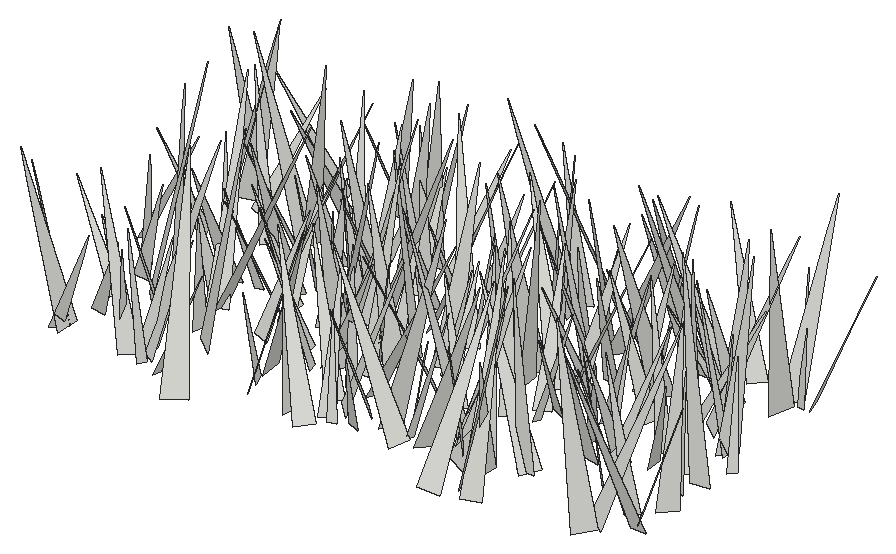
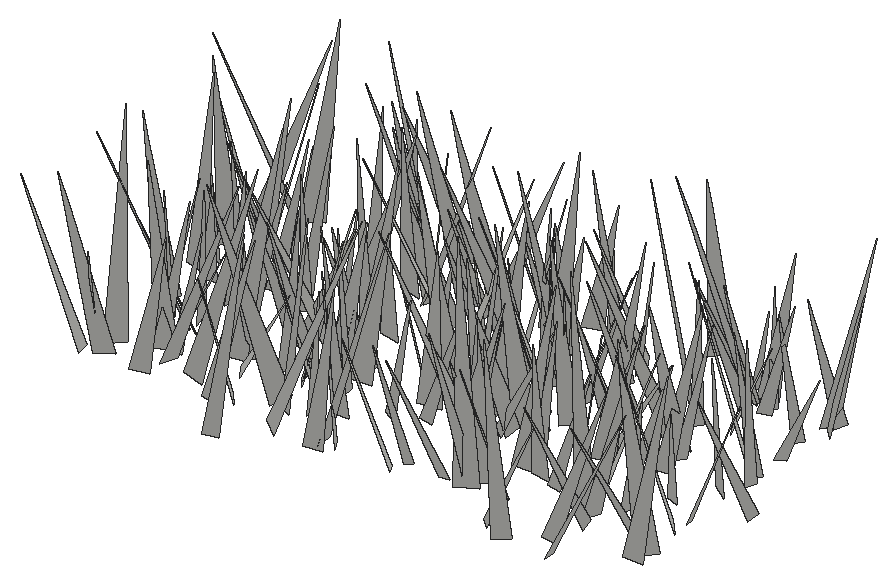
# SketchUp Ruby script. Lengths in inches.
U = 1.inch
M = Sketchup.active_model
def pt(a) = Geom::Point3d.new(a.map { |v| v * U })
def face(e, loops, mat)
  f = e.add_face(loops[0].map { |a| pt(a) })
  loops[1..].each { |l| e.add_face(l.map { |a| pt(a) }).erase! }
  f.material = f.back_material = mat if mat
  f
end
# faces: each face lists its corners as indices into pts; further lists are holes
def faces(e, pts, list, mat = nil) = list.each { |f| face(e, (f[0].is_a?(Array) ? f : [f]).map { |l| l.map { |i| pts[i] } }, mat) }
# xy, xz, yz: faces in a plane at the given z, y or x. An outline is a flat list of corners, or four numbers for a rectangle; further outlines are holes
def ring(l) = l.size == 4 ? [[l[0], l[1]], [l[2], l[1]], [l[2], l[3]], [l[0], l[3]]] : l.each_slice(2).to_a
def flat(e, list, mat, &to3) = list.each { |f| face(e, (f[0].is_a?(Array) ? f : [f]).map { |l| ring(l).map { |u, v| to3.(u, v) } }, mat) }
def xy(e, z, list, mat = nil) = flat(e, list, mat) { |x, y| [x, y, z] }
def xz(e, y, list, mat = nil) = flat(e, list, mat) { |x, z| [x, y, z] }
def yz(e, x, list, mat = nil) = flat(e, list, mat) { |y, z| [x, y, z] }
def lines(e, pts, list) = list.each { |a, b| e.add_line(pt(pts[a]), pt(pts[b])) }
# prism: a flat outline (further loops are holes) pulled along v
def prism(e, loops, v, mat = nil)
  f = face(e, loops, mat); d = Geom::Vector3d.new(v.map { |x| x * U })
  f.pushpull(f.normal.samedirection?(d) ? d.length : -d.length)
end
def box(e, o, s, mat = nil) = prism(e, [[o, [o[0] + s[0], o[1], o[2]], [o[0] + s[0], o[1] + s[1], o[2]], [o[0], o[1] + s[1], o[2]]]], [0, 0, s[2]], mat)
def at(x, y, z, deg = 0) = Geom::Transformation.translation(pt([x, y, z])) * Geom::Transformation.rotation(ORIGIN, Z_AXIS, deg.degrees)
def axes(o, x, y, z) = Geom::Transformation.new([*x, 0, *y, 0, *z, 0, *pt(o).to_a, 1])
def part(name) = M.definitions.add(name)
# library, detail: a bought-in or finely detailed component or shape, given as its bounding box
def library(name, o, s) = part(name).tap { |d| box(d.entities, o, s) }
def detail(e, o, s) = box(e.add_group.entities, o, s)
def put(e, d, t, mat = nil) = e.add_instance(d, t).tap { |i| i.material = mat if mat }
def group(e, t, mat = nil) = e.add_group.tap { |g| g.transformation = t; g.material = mat if mat }.entities
root = M.entities
c1 = part("fur_instance\#9")
p = [[0.8125,0,1.79],[0.67,-0.02,1.48],[0,-0.11,0],[0,0.11,0]]
faces(c1.entities,p,[[0,1,2,3]])
put(root,c1,axes([504.47,355.8125,-21.66],[-6.49711,1.14641,2.18071],[1.63194,6.61021,1.38712],[1.84567,-1.80917,6.45001]))
put(root,c1,axes([515.51,352.76,-21.66],[-5.56313,6.05819,1.00831],[6.02083,5.64819,-0.71719],[1.2116,-0.25113,8.19364]))
put(root,c1,axes([503.92,355.33,-21.66],[3.45367,-2.54495,0.42724],[-2.57712,-3.36456,0.79082],[0.1334,0.88889,4.21654]))
put(root,c1,axes([546.35,355.52,-21.66],[-5.45216,4.70878,2.71596],[5.23215,5.58914,0.81316],[1.47433,-2.42158,7.15803]))
put(root,c1,axes([512.55,354.71,-21.66],[3.9235,0.14114,0.37721],[0.06723,-3.8717,0.74932],[-0.3971,0.73898,3.85386]))
put(root,c1,axes([508.625,356.28,-21.66],[3.85883,-1.0172,1.02296],[-0.87371,-3.97244,-0.65425],[-1.14794,-0.39587,3.93665]))
put(root,c1,axes([526.52,357.02,-21.66],[-0.43336,-3.79274,0.22877],[-3.61563,0.48241,1.14868],[1.16807,0.08612,3.64049]))
put(root,c1,axes([536.4,355.625,-21.66],[7.04246,3.4796,1.7186],[3.70112,-7.09298,-0.80545],[-1.16744,-1.49647,7.81378]))
put(root,c1,axes([509.68,355.46,-21.66],[-3.34146,5.15286,1.47209],[5.35695,3.16362,1.08579],[-0.14849,-1.82317,6.0447]))
put(root,c1,axes([535.42,353.48,-21.66],[-1.59566,7.05244,0.57454],[6.94745,1.67322,-1.24356],[1.34162,-0.27674,7.12297]))
put(root,c1,axes([548.9,357.82,-21.66],[-1.75901,-6.72397,0.92553],[-6.70142,1.56883,-1.33876],[-1.07676,1.22044,6.82009]))
put(root,c1,axes([510.99,355.13,-21.66],[-4.31173,0.11749,0.33288],[0.02447,4.16916,-1.1546],[0.35215,1.14887,4.15592]))
put(root,c1,axes([504.12,356.31,-21.66],[-4.01169,-3.78695,1.3287],[-4.00574,3.89344,-0.9976],[0.2459,1.64323,5.42581]))
put(root,c1,axes([536.8,357.75,-21.66],[4.83805,-1.95602,0.87332],[-1.75837,-4.85831,-1.14034],[-1.22345,-0.75248,5.09238]))
put(root,c1,axes([522.14,355.82,-21.66],[-3.8319,-0.08961,1.0116],[-0.27638,3.8917,-0.7022],[0.97723,0.7493,3.76807]))
put(root,c1,axes([524.01,355.26,-21.66],[-3.78417,5.30239,0.2634],[5.25954,3.70033,1.07214],[-0.72248,-0.83479,6.42541]))
put(root,c1,axes([510.1875,356.3125,-21.66],[0.83525,-3.69964,2.10924],[-4.22949,-0.46947,0.8514],[0.49764,2.21949,3.69595]))
put(root,c1,axes([508.67,357.04,-21.66],[-2.76713,3.18046,1.2921],[3.43249,2.58898,0.97827],[0.05304,-1.61979,4.10065]))
put(root,c1,axes([534.81,357.94,-21.66],[3.60771,1.96245,2.32029],[2.67745,-3.75626,-0.98607],[-1.43745,-2.07119,3.98679]))
put(root,c1,axes([518.16,357.95,-21.66],[-3.2792,-1.26365,1.37089],[-0.97388,3.52607,0.9207],[1.58988,-0.44645,3.3915]))
put(root,c1,axes([530.21,357.05,-21.66],[-6.66331,2.16551,0.21128],[2.17487,6.60915,0.85019],[-0.06344,-0.87375,6.95459]))
put(root,c1,axes([526.24,359.1,-21.66],[-3.04266,-3.74721,0.50143],[-3.60797,3.07034,1.05183],[1.12942,-0.28668,4.71094]))
put(root,c1,axes([538.24,354.21,-21.66],[0.0768,8.17284,0.16546],[8.06568,-0.10268,1.32775],[-1.3295,-0.15078,8.06464]))
put(root,c1,axes([510.43,356.23,-21.66],[4.03025,7.20792,1.49357],[7.34455,-3.82368,-1.36555],[0.49235,-1.96292,8.14446]))
put(root,c1,axes([504.72,358.59,-21.66],[1.3305,-3.93215,0.09517],[-3.71952,-1.22514,1.38031],[1.27907,0.52755,3.91494]))
put(root,c1,axes([531.71,357.85,-21.66],[6.48225,-3.39085,0.68777],[-3.4557,-6.41712,0.9323],[-0.17042,1.14593,7.25591]))
put(root,c1,axes([525.15,356.56,-21.66],[-0.19051,3.61425,0.52762],[3.57644,0.0773,0.76192],[-0.74175,-0.55561,3.53816]))
put(root,c1,axes([534.33,357.69,-21.66],[1.01992,4.1189,1.46608],[4.23417,-0.55549,-1.38501],[1.0893,-1.69737,4.0109]))
put(root,c1,axes([510.3,357.03,-21.66],[3.86814,-0.78573,1.02615],[-1.07279,-3.75781,1.16655],[-0.72076,1.37634,3.77081]))
put(root,c1,axes([546.43,359.55,-21.66],[-4.48519,-3.52054,0.94744],[-3.42145,4.58335,0.83384],[1.25916,-0.08621,5.64055]))
put(root,c1,axes([518.52,356.51,-21.66],[4.75922,3.00167,0.77273],[2.8511,-4.79497,1.06623],[-1.21588,0.50555,5.5248]))
put(root,c1,axes([517.86,359.57,-21.66],[6.9866,-0.46387,0.39437],[-0.38095,-6.874,-1.33651],[-0.47495,-1.31005,6.87325]))
put(root,c1,axes([524.48,356.93,-21.66],[-3.96377,3.38106,0.80717],[3.27975,4.04327,-0.83051],[1.15166,0.12228,5.14327]))
put(root,c1,axes([533.98,358.76,-21.66],[4.85202,-3.37562,1.03104],[-3.52041,-4.75453,1.00059],[-0.25408,1.41409,5.82544]))
put(root,c1,axes([546.23,356.82,-21.66],[3.64323,6.95762,0.66244],[6.95502,-3.53547,-1.11744],[0.68929,-1.10109,7.77386]))
put(root,c1,axes([548.1,359.01,-21.66],[4.88732,1.92922,0.49219],[1.99044,-4.76555,-1.08522],[-0.04774,-1.19066,5.14102]))
put(root,c1,axes([524.73,358.3125,-21.66],[4.20289,4.66758,0.96744],[4.74909,-3.98911,-1.38552],[0.41036,-1.63927,6.12625]))
put(root,c1,axes([534.64,357.26,-21.66],[3.51205,7.24819,1.1392],[7.33442,-3.43356,-0.76524],[0.20101,-1.35755,8.01781]))
put(root,c1,axes([534.61,358.64,-21.66],[-7.94923,-1.56442,0.5472],[-1.62855,7.87073,-1.15603],[0.30767,1.24144,8.0188]))
put(root,c1,axes([547.24,359.23,-21.66],[0.3865,-5.10308,2.42648],[-5.49086,-0.91339,-1.04632],[-1.33405,2.28099,5.00959]))
put(root,c1,axes([529.2,359.67,-21.66],[3.2608,1.42212,0.87051],[1.60342,-3.19897,-0.78016],[-0.45742,-1.07574,3.47082]))
put(root,c1,axes([530.23,358.1,-21.66],[4.26964,0.47793,1.18834],[0.14194,-4.28676,1.21405],[-1.27296,1.12502,4.1212]))
put(root,c1,axes([528.43,358.43,-21.66],[7.3545,-2.24014,2.18394],[-2.66673,-7.40612,1.38362],[-1.63595,2.00191,7.56257]))
put(root,c1,axes([538.65,359.22,-21.66],[-1.16984,-6.03511,2.92768],[-6.70455,0.96018,-0.69968],[-0.2073,3.00298,6.1075]))
put(root,c1,axes([538.87,359.4,-21.66],[-5.22041,4.31379,0.87725],[4.39805,5.05275,1.32586],[-0.18846,-1.57859,6.64105]))
put(root,c1,axes([512.71,359.26,-21.66],[4.94057,6.27292,2.28459],[6.62263,-4.9638,-0.69253],[-0.84236,-2.23369,7.95482]))
put(root,c1,axes([511.12,360.8125,-21.66],[4.3252,-1.84495,1.08949],[-1.74272,-4.45705,-0.62914],[-1.2465,-0.1704,4.65998]))
put(root,c1,axes([523.49,358.92,-21.66],[-3.54308,4.52564,0.44169],[4.5332,3.47169,0.79207],[-0.35583,-0.83417,5.69276]))
put(root,c1,axes([544.8,359.54,-21.66],[-3.71707,-2.68533,1.32909],[-2.9797,3.53518,-1.19076],[0.31439,1.75658,4.42828]))
put(root,c1,axes([509.03,359.91,-21.66],[-3.56795,-1.90054,0.20659],[-1.88749,3.43261,-1.0196],[-0.30353,0.99505,3.91187]))
put(root,c1,axes([535.87,358.77,-21.66],[0.42916,7.00561,1.64499],[7.11073,-0.66598,0.98114],[-1.10544,-1.56418,6.94983]))
put(root,c1,axes([521.37,362.57,-21.66],[4.41778,-6.32124,1.65754],[-6.32459,-4.6393,-0.83587],[-1.6447,0.86086,7.66656]))
put(root,c1,axes([540.92,362.95,-21.66],[-0.50575,-5.47671,0.42869],[-5.44927,0.55465,0.65709],[0.69543,0.36321,5.46062]))
put(root,c1,axes([504.24,361.02,-21.66],[-3.16167,2.60611,0.16715],[2.5519,3.02748,1.0668],[-0.55458,-0.92652,3.956]))
put(root,c1,axes([527.65,364.02,-21.66],[-3.98509,-5.15803,0.00595],[-5.07141,3.91953,1.18509],[0.94137,-0.71992,6.40951]))
put(root,c1,axes([519.8,361.34,-21.66],[-5.05494,-2.22544,0.30278],[-2.23904,4.935,-1.10864],[-0.17591,1.1357,5.41072]))
put(root,c1,axes([525.05,361,-21.66],[6.85637,-0.90607,0.05149],[-0.90407,-6.7849,0.99057],[0.07926,0.98874,6.84468]))
put(root,c1,axes([548.83,360.82,-21.66],[5.64429,-3.09602,3.33103],[-3.78051,-6.14532,0.69416],[-2.52761,2.27789,6.40012]))
put(root,c1,axes([520.56,362.1,-21.66],[4.45339,-2.56263,0.11815],[-2.55046,-4.39735,0.75645],[0.27609,0.71411,5.08208]))
put(root,c1,axes([518.36,362.95,-21.66],[-4.47409,-0.55232,0.95951],[-0.288,4.43762,1.21151],[1.069,-1.11608,4.34221]))
put(root,c1,axes([521.87,363.01,-21.66],[-2.90046,-3.39812,1.38689],[-3.27993,3.19309,0.96417],[1.64705,0.37459,4.36237]))
put(root,c1,axes([523.17,361.1,-21.66],[-4.45117,0.87592,1.04433],[0.68712,4.52233,-0.86441],[1.17717,0.67238,4.45342]))
put(root,c1,axes([542.72,363.91,-21.66],[2.25117,-4.50739,0.41367],[-4.42833,-2.28883,-0.84056],[-0.93676,-0.01195,4.96767]))
put(root,c1,axes([530.92,360.55,-21.66],[-2.87102,4.68172,0.40163],[4.57171,2.89185,-1.02921],[1.08596,0.20316,5.39463]))
put(root,c1,axes([504.1,363.71,-21.66],[1.4923,-4.43759,0.64343],[-4.35505,-1.27294,1.3215],[1.06759,1.01025,4.49142]))
put(root,c1,axes([521.22,361.35,-21.66],[7.46967,2.68884,2.29218],[2.3982,-7.79505,1.32883],[-2.59473,0.53597,7.82688]))
put(root,c1,axes([514.8,362.32,-21.66],[0.90877,4.85728,1.17196],[4.86719,-0.59112,-1.32422],[1.13009,-1.36012,4.76083]))
put(root,c1,axes([539.5,364.69,-21.66],[4.03439,-1.67825,0.01541],[-1.64329,-3.95818,-0.85174],[-0.3411,-0.78061,4.28572]))
put(root,c1,axes([544.43,364.96,-21.66],[4.66467,-0.77947,0.02704],[-0.7406,-4.47818,-1.32848],[-0.24456,-1.30606,4.53893]))
put(root,c1,axes([522.87,364.08,-21.66],[4.02483,1.17033,1.17041],[1.40502,-4.04247,-0.78939],[-0.87491,-1.10794,4.11653]))
put(root,c1,axes([542.56,362.9,-21.66],[2.02103,5.13059,0.73898],[5.12624,-1.86067,-1.10143],[0.76856,-1.08099,5.40318]))
put(root,c1,axes([503.64,364.75,-21.66],[4.65785,-0.69082,1.21899],[-0.53967,-4.78978,-0.65231],[-1.29303,-0.48941,4.6634]))
put(root,c1,axes([547.98,363.13,-21.66],[1.43677,3.63281,1.03111],[3.57622,-1.66329,0.8769],[-1.21291,-0.60083,3.80693]))
put(root,c1,axes([523.82,364.66,-21.66],[4.51203,-4.20905,2.90182],[-4.30887,-5.21386,-0.8628],[-2.75143,1.26279,6.10984]))
put(root,c1,axes([509.2,364.93,-21.66],[-4.57691,0.82768,1.57562],[1.18388,4.66198,0.99001],[1.32893,-1.30255,4.54457]))
put(root,c1,axes([530.36,363.13,-21.66],[-1.14245,4.14217,0.46464],[4.01441,0.96381,1.27839],[-1.12161,-0.76952,4.10226]))
put(root,c1,axes([530.07,361.83,-21.66],[5.64336,5.1887,0.30355],[5.15395,-5.64438,0.66329],[-0.67191,0.28398,7.63742]))
put(root,c1,axes([506.14,362.1,-21.66],[-5.10797,-4.03263,5.02727],[-5.71036,5.80586,-1.14484],[2.98787,4.202,6.40647]))
put(root,c1,axes([519.36,363.625,-21.66],[-4.01098,-1.65554,1.8183],[-2.11594,4.09606,-0.93811],[1.25294,1.61753,4.23659]))
put(root,c1,axes([509.04,366.8,-21.66],[1.9027,-5.40071,0.1352],[-5.35593,-1.9045,-0.70218],[-0.70705,-0.10684,5.68285]))
put(root,c1,axes([535.49,366.47,-21.66],[-0.82646,-4.24361,0.01629],[-4.06802,0.79698,1.2278],[1.20816,-0.21938,4.14533]))
put(root,c1,axes([519.57,365.82,-21.66],[4.8829,2.83209,2.83107],[3.60518,-5.05239,-1.16384],[-1.7431,-2.51617,5.52349]))
put(root,c1,axes([510.49,363.76,-21.66],[7.61599,0.93725,0.32253],[0.89381,-7.57423,0.90437],[-0.42844,0.85927,7.61996]))
put(root,c1,axes([523.23,362.58,-21.66],[1.19903,6.87384,0.5978],[6.78552,-1.2847,1.16229],[-1.25048,-0.38022,6.88014]))
put(root,c1,axes([517.38,365.77,-21.66],[3.13574,-5.33007,1.5739],[-5.55752,-3.01682,0.85589],[-0.02918,1.79133,6.12454]))
put(root,c1,axes([548.32,364.73,-21.66],[-0.94907,-6.99906,3.73248],[-7.88487,0.42284,-1.21201],[-0.8643,3.82797,6.95835]))
put(root,c1,axes([527.21,365.42,-21.66],[1.77196,3.84512,1.4323],[4.08534,-1.50774,-1.0065],[0.38272,-1.70823,4.11239]))
put(root,c1,axes([513.53,365.76,-21.66],[-2.7685,-2.84273,0.0732],[-2.6967,2.59213,-1.32656],[-0.90237,0.97511,3.73978]))
put(root,c1,axes([512.94,368.01,-21.66],[2.89826,-6.60565,0.55734],[-6.55377,-2.94663,-0.84295],[-0.99662,0.16719,7.16407]))
put(root,c1,axes([513.47,364.89,-21.66],[4.56915,3.9518,0.34933],[3.96081,-4.51383,-0.74378],[0.22516,-0.79028,5.99505]))
put(root,c1,axes([533.29,364.11,-21.66],[-0.40472,6.25604,0.83945],[6.18781,0.22712,1.29072],[-1.24649,-0.90382,6.13481]))
put(root,c1,axes([535.0625,364.87,-21.66],[3.77133,0.16267,0.95437],[-0.10228,-3.74984,1.04331],[-0.96272,1.03561,3.6278]))
put(root,c1,axes([514.96,364.61,-21.66],[-0.69382,4.82103,0.91338],[4.82167,0.84094,-0.77604],[0.90996,-0.78004,4.80848]))
put(root,c1,axes([514.3125,366.68,-21.66],[-4.64353,0.24048,0.81476],[0.40253,4.60984,0.93348],[0.74809,-0.98772,4.55508]))
put(root,c1,axes([541.4375,364.29,-21.66],[1.45734,4.18221,0.34787],[4.02467,-1.49715,1.13854],[-1.18907,0.05834,4.28]))
put(root,c1,axes([510.81,367.19,-21.66],[-0.75955,-3.70224,0.74684],[-3.72635,0.61048,-0.76351],[-0.61539,0.87293,3.70143]))
put(root,c1,axes([510.29,363.62,-21.66],[-0.64935,7.68845,0.01437],[7.6155,0.6412,1.06165],[-1.05669,-0.10353,7.64243]))
put(root,c1,axes([546.79,365.46,-21.66],[-1.86757,4.60063,0.33127],[4.58089,1.80817,0.71369],[-0.53944,-0.57279,4.91369]))
put(root,c1,axes([524.35,366.22,-21.66],[-6.69372,-1.63538,1.73187],[-1.91789,6.76382,-1.02573],[1.41263,1.43387,6.81383]))
put(root,c1,axes([520.12,364.43,-21.66],[5.47327,5.90798,0.9862],[5.7796,-5.55993,1.23167],[-1.57262,0.12835,7.95889]))
put(root,c1,axes([526.42,366.43,-21.66],[-2.68799,6.56885,2.98447],[6.8694,3.30396,-1.08507],[2.20641,-2.2839,7.01411]))
put(root,c1,axes([518.26,366.83,-21.66],[4.16572,3.95636,0.93283],[4.06431,-4.03236,-1.04767],[0.06588,-1.40123,5.64875]))
put(root,c1,axes([531.66,368.18,-21.66],[7.52805,-0.18805,1.99939],[0.07054,-7.72753,-0.99239],[-2.00698,-0.97696,7.46472]))
put(root,c1,axes([543.89,366.61,-21.66],[-5.59826,1.4556,0.99849],[1.35798,5.67289,-0.65612],[1.12768,0.39476,5.74707]))
put(root,c1,axes([537,368.57,-21.66],[-0.83843,-4.56243,0.7415],[-4.45874,0.59959,-1.35228],[-1.2187,0.94513,4.43735]))
put(root,c1,axes([534.55,366.07,-21.66],[-3.134,4.47853,0.59876],[4.43295,3.18866,-0.64743],[0.8745,-0.1137,5.42771]))
put(root,c1,axes([504.61,366.59,-21.66],[2.34142,5.16985,1.64131],[5.10687,-2.70355,1.23051],[-1.82787,-0.93109,5.54034]))
put(root,c1,axes([519.28,367.85,-21.66],[3.63637,-5.76719,3.12725],[-6.51934,-3.57646,0.98508],[-0.73369,3.19558,6.74635]))
put(root,c1,axes([548.88,367.28,-21.66],[-3.45785,1.40655,0.59459],[1.25916,3.45892,-0.85969],[0.86397,0.58836,3.63264]))
put(root,c1,axes([531.18,369.7,-21.66],[1.42395,-7.42701,2.10024],[-7.62151,-1.69014,-0.80943],[-1.21824,1.89264,7.51884]))
put(root,c1,axes([540.77,369.17,-21.66],[4.1746,-2.61988,2.8232],[-2.37692,-5.02847,-1.15163],[-3.03059,0.33503,4.79215]))
put(root,c1,axes([500.97,367.82,-21.66],[4.26787,-0.90452,0.30078],[-0.95208,-4.11231,1.14272],[-0.04649,1.18073,4.21035]))
put(root,c1,axes([538.54,367.42,-21.66],[5.15508,0.33774,1.32609],[0.02228,-5.18864,1.23487],[-1.36825,1.188,5.01637]))
put(root,c1,axes([520.3125,369.32,-21.66],[-2.43952,-3.83837,0.4143],[-3.75379,2.24378,-1.31547],[-0.90209,1.04325,4.3536]))
put(root,c1,axes([513.32,369.81,-21.66],[-3.34648,-2.86729,1.25208],[-2.75468,3.56945,0.81158],[1.4835,0.16004,4.33146]))
put(root,c1,axes([527.27,367.9,-21.66],[2.58432,3.47984,0.90101],[3.42396,-2.72089,0.68775],[-1.09434,-0.29537,4.2796]))
put(root,c1,axes([535.36,367.34,-21.66],[6.4283,2.09347,0.22673],[2.03253,-6.35917,1.08941],[-0.55031,0.96716,6.67224]))
put(root,c1,axes([521.74,367.5,-21.66],[-3.54385,2.2292,0.7922],[1.93522,3.55225,-1.33876],[1.36083,0.75365,3.96686]))
put(root,c1,axes([503.71,370.86,-21.66],[-4.07009,-1.55263,0.42821],[-1.43545,4.0247,0.94922],[0.73043,-0.7422,4.25151]))
put(root,c1,axes([547.19,368.84,-21.66],[-5.62081,-1.07857,0.79033],[-1.22962,5.511,-1.22409],[0.52534,1.35906,5.59093]))
put(root,c1,axes([519.67,368.57,-21.66],[7.1879,-0.3196,1.18159],[-0.53762,-7.14753,1.33717],[-1.09967,1.40532,7.06966]))
put(root,c1,axes([547.17,368.96,-21.66],[-5.57842,3.33095,2.99608],[3.28064,6.29556,-0.89096],[3.05108,-0.67911,6.43585]))
put(root,c1,axes([535.6875,371.54,-21.66],[0.34868,-5.31048,0.36463],[-5.26358,-0.28954,0.81646],[0.79301,0.41316,5.25892]))
put(root,c1,axes([539.31,372.23,-21.66],[2.6009,-7.25193,0.96085],[-7.2129,-2.71231,-0.94648],[-1.21974,0.57558,7.64587]))
put(root,c1,axes([516.49,370.0625,-21.66],[0.55696,-4.64877,2.01019],[-4.98122,-0.86859,-0.62855],[-0.91614,1.89648,4.63963]))
put(root,c1,axes([524.76,371.05,-21.66],[0.09538,-4.31944,0.7575],[-4.29634,-0.24392,-0.84995],[-0.8791,0.72346,4.23607]))
put(root,c1,axes([545.83,370.31,-21.66],[-1.72893,-3.46771,1.76985],[-3.62718,2.13831,0.64633],[1.41454,1.24466,3.82053]))
put(root,c1,axes([533.6,368.9,-21.66],[-4.22823,5.63878,0.60494],[5.64653,4.11564,1.10357],[-0.52773,-1.14251,6.96102]))
put(root,c1,axes([534,372.06,-21.66],[-4.57132,-4.01454,0.83204],[-3.89365,4.6413,1.00178],[1.28384,-0.21818,6.00082]))
put(root,c1,axes([506.25,369.35,-21.66],[0.5097,3.85536,0.87755],[3.83119,-0.70034,0.85159],[-0.9777,-0.73445,3.79452]))
put(root,c1,axes([509.72,372.45,-21.66],[-3.92471,-3.72483,0.22437],[-3.66233,3.90735,0.80501],[0.71557,-0.43166,5.35067]))
put(root,c1,axes([530.95,371.2,-21.66],[5.21956,1.10973,1.69595],[1.36173,-5.39042,-0.66376],[-1.50115,-1.03121,5.29478]))
put(root,c1,axes([543.97,369.72,-21.66],[-5.50715,-0.70612,1.61288],[-1.08889,5.52799,-1.29784],[1.38358,1.53996,5.39842]))
put(root,c1,axes([516.32,371.95,-21.66],[1.47343,-6.07806,1.78682],[-6.21699,-1.74005,-0.79238],[-1.21846,1.52838,6.20371]))
put(root,c1,axes([521.0625,372.125,-21.66],[-0.49716,-5.04462,0.80589],[-5.07325,0.39247,-0.67299],[-0.59982,0.86174,5.02418]))
put(root,c1,axes([525.83,369.39,-21.66],[-2.86004,7.00076,0.77945],[7.00763,2.7424,1.08181],[-0.71502,-1.12544,7.48466]))
put(root,c1,axes([522.47,369.97,-21.66],[7.12948,2.21776,0.41944],[2.17259,-7.11974,0.71624],[-0.61174,0.56098,7.43203]))
put(root,c1,axes([533.8125,370.84,-21.66],[0.03547,5.69131,1.501],[5.73382,0.30561,-1.29426],[1.32938,-1.46999,5.5423]))
put(root,c1,axes([534.32,371.07,-21.66],[-6.24639,-1.28271,0.8155],[-1.43317,6.11916,-1.35263],[0.50635,1.49608,6.23162]))
put(root,c1,axes([513.14,372.71,-21.66],[0.25989,-4.12749,1.06746],[-4.12688,-0.51192,-0.97467],[-1.06982,0.97209,4.01917]))
put(root,c1,axes([538.07,371.49,-21.66],[0.29151,4.89673,1.62599],[5.06271,0.04273,-1.03633],[0.99541,-1.65136,4.79468]))
put(root,c1,axes([542.84,371.53,-21.66],[3.55975,3.91646,0.08522],[3.79537,-3.41954,-1.38552],[0.97011,-0.99289,5.10792]))
put(root,c1,axes([531.6,371.91,-21.66],[-3.37291,-1.64413,0.77782],[-1.79286,3.28135,-0.83849],[0.30629,1.10194,3.65741]))
put(root,c1,axes([509.95,373.53,-21.66],[7.47084,-2.00529,1.5784],[-1.88161,-7.62701,-0.78379],[-1.72397,-0.36551,7.69548]))
put(root,c1,axes([544.35,370.73,-21.66],[4.64022,6.0526,0.40907],[6.0581,-4.59639,-0.71102],[0.31728,-0.75645,7.59342]))
put(root,c1,axes([526.85,372.03,-21.66],[-2.00481,-4.221,2.16779],[-4.72189,1.54205,-1.3643],[-0.46899,2.51807,4.46932]))
put(root,c1,axes([542.77,374.26,-21.66],[-3.89152,-1.38284,0.09587],[-1.31779,3.77936,1.02238],[0.42995,-0.93252,4.00136]))
put(root,c1,axes([543.67,374.25,-21.66],[3.33283,-3.55166,1.19436],[-3.37517,-3.53973,-1.10774],[-1.62758,0.06765,4.74288]))
put(root,c1,axes([533.24,371.87,-21.66],[3.40494,2.47984,0.75094],[2.39973,-3.48584,0.63038],[-0.97714,0.08048,4.16483]))
put(root,c1,axes([542.47,374.17,-21.66],[-3.58815,0.95471,1.93369],[1.59157,3.70529,1.12394],[1.45517,-1.69849,3.5388]))
put(root,c1,axes([519.88,372.61,-21.66],[-5.84783,-0.54956,0.92386],[-0.66437,5.86496,-0.71656],[0.84507,0.80798,5.82972]))
put(root,c1,axes([537.84,373.4375,-21.66],[-3.22375,-2.36609,0.00506],[-2.25529,3.0702,-1.21594],[-0.71558,0.9831,3.80952]))
put(root,c1,axes([529.29,373.86,-21.66],[-0.7765,-5.95979,2.50914],[-6.25232,1.3369,1.24057],[1.65027,2.26084,5.88073]))
put(root,c1,axes([509.01,374.1,-21.66],[-7.26017,0.65472,1.63239],[0.85,7.37598,0.82207],[1.53976,-0.9847,7.24313]))
put(root,c1,axes([507.7,372.04,-21.66],[-5.44212,1.96061,0.21811],[1.90755,5.39324,-0.88463],[0.50284,0.7598,5.71648]))
put(root,c1,axes([519.85,372.75,-21.66],[-5.54219,0.95074,1.40051],[0.80502,5.69802,-0.68242],[1.48905,0.4581,5.58158]))
put(root,c1,axes([514.65,372.1875,-21.66],[-0.46142,6.00885,1.03301],[6.04976,0.32253,0.82618],[-0.75742,-1.08443,5.96964]))
put(root,c1,axes([543.51,373.78,-21.66],[3.4619,-5.09824,2.22403],[-5.52391,-3.4582,0.67108],[-0.65172,2.22978,6.12588]))
put(root,c1,axes([546.36,375.39,-21.66],[6.94101,-3.43299,1.84422],[-3.2352,-7.17632,-1.18245],[-2.17258,-0.28153,7.65277]))
put(root,c1,axes([516.83,374.8,-21.66],[2.07554,-6.96607,1.71735],[-7.11885,-1.77704,1.39545],[0.89291,2.02467,7.13349]))
put(root,c1,axes([532.55,375.59,-21.66],[-2.91514,-5.53327,1.42514],[-5.42873,3.18122,1.24695],[1.78243,0.63944,6.12864]))
put(root,c1,axes([530.92,374.85,-21.66],[3.87563,-0.57439,1.14349],[-0.32332,-3.96837,-0.89752],[-1.23813,-0.76168,3.81378]))
put(root,c1,axes([504.06,371.9375,-21.66],[5.15399,5.0376,1.12923],[4.93282,-5.27609,1.02292],[-1.5231,-0.04087,7.13405]))
put(root,c1,axes([519.14,372.74,-21.66],[-2.23012,3.65012,0.738],[3.54975,2.34365,-0.86487],[1.12574,-0.15918,4.18913]))
put(root,c1,axes([539.7,375.89,-21.66],[-1.24664,-7.42641,1.30497],[-7.49381,1.07378,-1.04811],[-0.83512,1.45053,7.45702]))
put(root,c1,axes([542.29,375.07,-21.66],[-7.15146,0.58689,0.88826],[0.71619,7.11549,1.06478],[0.78773,-1.14116,7.09606]))
put(root,c1,axes([533.6,374.65,-21.66],[7.07032,-2.50038,0.22823],[-2.5064,-6.98854,1.08245],[0.14815,1.09629,7.42089]))
put(root,c1,axes([517.47,376.125,-21.66],[3.37968,-7.43588,1.46776],[-7.57694,-3.27406,0.85991],[0.19143,1.6903,8.12251]))
put(root,c1,axes([503.16,375.76,-21.66],[4.2743,-5.66959,1.70794],[-5.91958,-4.14155,1.06631],[-0.14077,2.00854,7.01974]))
put(root,c1,axes([503.41,376.9,-21.66],[0.65749,-6.30029,1.7132],[-6.47052,-0.85883,-0.67511],[-0.87239,1.62165,6.29842]))
put(root,c1,axes([514.63,375.6,-21.66],[2.82445,3.52777,0.66946],[3.53756,-2.58781,-1.2883],[0.61561,-1.31488,4.33162]))
put(root,c1,axes([531.93,377.8,-21.66],[-4.63636,-6.55031,0.51962],[-6.56307,4.58532,-0.75728],[-0.32055,0.86066,7.9893]))
put(root,c1,axes([509.1,378.15,-21.66],[0.9036,-5.03288,0.01557],[-4.93923,-0.88981,-0.97923],[-0.96652,-0.158,5.01871]))
put(root,c1,axes([528.16,377.11,-21.66],[-7.66466,-1.90179,1.421],[-1.79066,7.78455,0.75987],[1.55871,-0.40873,7.86043]))
put(root,c1,axes([537.15,377.46,-21.66],[-0.33805,-5.61743,0.95415],[-5.65981,0.22074,-0.70569],[-0.6576,0.9879,5.58317]))
put(root,c1,axes([522.22,375.98,-21.66],[0.51441,-3.71167,1.78135],[-3.92489,0.09986,1.3415],[1.24297,1.85145,3.49879]))
put(root,c1,axes([504.625,374.74,-21.66],[1.15422,4.7345,0.08294],[4.6056,-1.10261,-1.15208],[1.10037,-0.35121,4.73502]))
put(root,c1,axes([508.52,375.2,-21.66],[4.79219,0.94532,0.41054],[0.81575,-4.67249,1.23678],[-0.62985,1.14081,4.72537]))
put(root,c1,axes([517.87,375.21,-21.66],[5.65388,1.0827,1.74004],[0.6959,-5.81697,1.3583],[-1.92762,1.07564,5.59407]))
put(root,c1,axes([527.24,377.0625,-21.66],[4.80931,3.10321,2.02961],[3.46778,-4.94111,-0.66234],[-1.31293,-1.68352,5.68513]))
put(root,c1,axes([547.49,377.28,-21.66],[5.84375,1.80801,0.13219],[1.81029,-5.79638,-0.74876],[0.09603,-0.75425,6.07105]))
put(root,c1,axes([519.3,376.07,-21.66],[0.97735,4.73028,0.44464],[4.65378,-0.86171,-1.06216],[0.95682,-0.64061,4.71196]))
put(root,c1,axes([522.7,377.19,-21.66],[4.03846,2.29721,0.25382],[2.30928,-3.98992,-0.63131],[0.09403,-0.6739,4.60302]))
put(root,c1,axes([547.07,376.47,-21.66],[1.77865,4.09096,1.0407],[3.89915,-2.02489,1.29578],[-1.61729,-0.38272,4.26855]))
put(root,c1,axes([536.0625,376.35,-21.66],[3.62964,3.56201,0.97293],[3.43547,-3.75775,0.94107],[-1.35352,0.01415,4.99765]))
put(root,c1,axes([528.16,378.22,-21.66],[1.39978,-5.30319,2.32473],[-5.64349,-1.78474,-0.67328],[-1.29585,2.04412,5.44334]))
put(root,c1,axes([542.875,377.3,-21.66],[-3.19469,4.99874,1.10839],[5.10889,3.02549,1.08057],[-0.33936,-1.5103,5.83317]))
put(root,c1,axes([507.88,379.77,-21.66],[-5.4355,-1.48683,0.1699],[-1.41481,5.31415,1.24191],[0.48767,-1.15472,5.49664]))
put(root,c1,axes([534.19,381,-21.66],[-0.43827,-6.52973,0.002],[-6.42899,0.43186,1.145],[1.14256,-0.07472,6.44348]))
put(root,c1,axes([513.7,378.92,-21.66],[-2.53875,-3.10556,0.31926],[-3.0835,2.42999,-0.88252],[-0.48832,0.80145,3.91291]))
put(root,c1,axes([546.03,376.91,-21.66],[-1.91497,6.86191,1.78883],[6.91485,2.21764,-1.10438],[1.57179,-1.39609,7.03799]))
put(root,c1,axes([511.66,379.85,-21.66],[2.30675,-6.01681,0.97122],[-6.03702,-2.11321,1.24701],[0.83643,1.34116,6.32203]))
